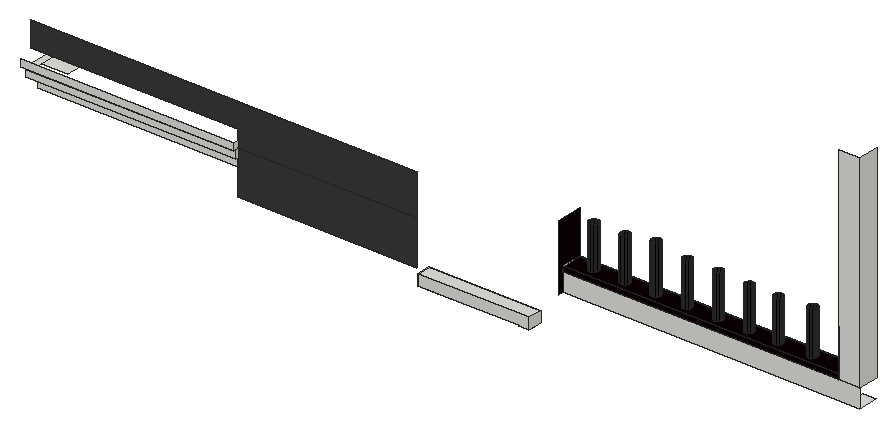
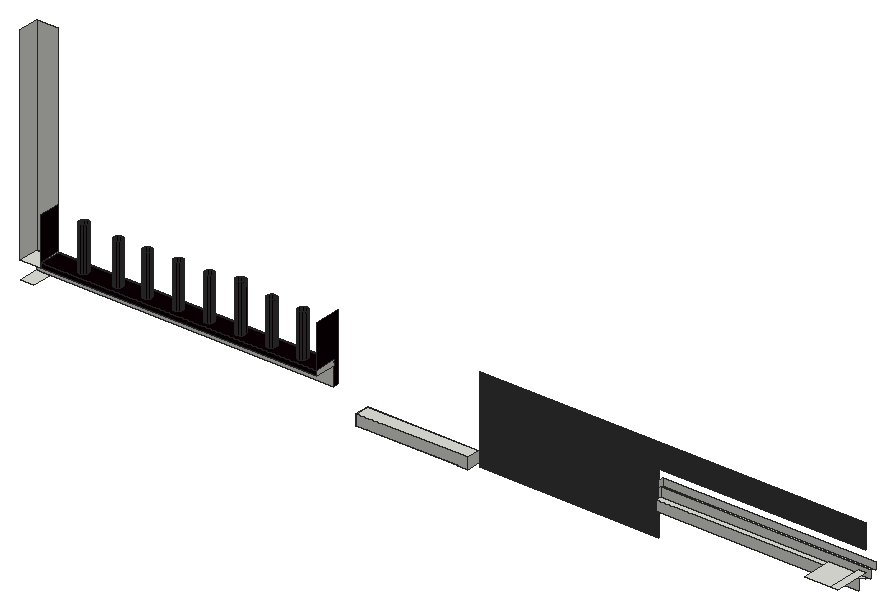
# SketchUp Ruby script. Lengths in inches.
U = 1.inch
M = Sketchup.active_model
def pt(a) = Geom::Point3d.new(a.map { |v| v * U })
def face(e, loops, mat)
  f = e.add_face(loops[0].map { |a| pt(a) })
  loops[1..].each { |l| e.add_face(l.map { |a| pt(a) }).erase! }
  f.material = f.back_material = mat if mat
  f
end
# faces: each face lists its corners as indices into pts; further lists are holes
def faces(e, pts, list, mat = nil) = list.each { |f| face(e, (f[0].is_a?(Array) ? f : [f]).map { |l| l.map { |i| pts[i] } }, mat) }
# xy, xz, yz: faces in a plane at the given z, y or x. An outline is a flat list of corners, or four numbers for a rectangle; further outlines are holes
def ring(l) = l.size == 4 ? [[l[0], l[1]], [l[2], l[1]], [l[2], l[3]], [l[0], l[3]]] : l.each_slice(2).to_a
def flat(e, list, mat, &to3) = list.each { |f| face(e, (f[0].is_a?(Array) ? f : [f]).map { |l| ring(l).map { |u, v| to3.(u, v) } }, mat) }
def xy(e, z, list, mat = nil) = flat(e, list, mat) { |x, y| [x, y, z] }
def xz(e, y, list, mat = nil) = flat(e, list, mat) { |x, z| [x, y, z] }
def yz(e, x, list, mat = nil) = flat(e, list, mat) { |y, z| [x, y, z] }
def lines(e, pts, list) = list.each { |a, b| e.add_line(pt(pts[a]), pt(pts[b])) }
# prism: a flat outline (further loops are holes) pulled along v
def prism(e, loops, v, mat = nil)
  f = face(e, loops, mat); d = Geom::Vector3d.new(v.map { |x| x * U })
  f.pushpull(f.normal.samedirection?(d) ? d.length : -d.length)
end
def box(e, o, s, mat = nil) = prism(e, [[o, [o[0] + s[0], o[1], o[2]], [o[0] + s[0], o[1] + s[1], o[2]], [o[0], o[1] + s[1], o[2]]]], [0, 0, s[2]], mat)
def at(x, y, z, deg = 0) = Geom::Transformation.translation(pt([x, y, z])) * Geom::Transformation.rotation(ORIGIN, Z_AXIS, deg.degrees)
def axes(o, x, y, z) = Geom::Transformation.new([*x, 0, *y, 0, *z, 0, *pt(o).to_a, 1])
def part(name) = M.definitions.add(name)
# library, detail: a bought-in or finely detailed component or shape, given as its bounding box
def library(name, o, s) = part(name).tap { |d| box(d.entities, o, s) }
def detail(e, o, s) = box(e.add_group.entities, o, s)
def put(e, d, t, mat = nil) = e.add_instance(d, t).tap { |i| i.material = mat if mat }
def group(e, t, mat = nil) = e.add_group.tap { |g| g.transformation = t; g.material = mat if mat }.entities
root = M.entities
M.materials.add("[Color M07]").color = [58, 58, 58]
M.materials.add("[Metal Seamed]").color = [11, 0, 4]
xy(root,387.29,[[283.95,58.1,290.34,67.28],[350.03,58.1,357.14,60.85],[291.14,60.85,350.03,67.28],[350.03,60.85,353.83,67.28],[353.83,60.85,357.14,67.28]])
xy(root,387.57,[[290.34,58.1,350.03,67.28]])
xy(root,394.6,[[283.95,58.1,357.14,67.28]])
xy(root,408,[[555.7,70.97,564.5,84.18]])
xy(root,414.75,[[21.75,65.66,21.75,67.28,24.25,67.28,24.25,69.47,158,69.47,158,65.66]])
xy(root,420,[[369.3125,70.97,550.8125,84.66],[550.8125,70.97,564.5,84.66]])
xy(root,420.5,[[21.75,63.91,158,65.66],[19.4375,70.02,24.07,92.83],[24.07,73.08,41.19,92.83]])
xy(root,423.375,[[383.69,75.15,382.92,75.25,382.19,75.55,381.57,76.03,381.09,76.65,380.79,77.37,380.69,78.15,380.79,78.92,381.09,79.65,381.57,80.27,382.19,80.75,382.92,81.05,383.69,81.15,384.47,81.05,385.19,80.75,385.8125,80.27,386.29,79.65,386.59,78.92,386.69,78.15,386.59,77.37,386.29,76.65,385.8125,76.03,385.19,75.55,384.47,75.25],[404.19,75.15,403.42,75.25,402.69,75.55,402.07,76.03,401.59,76.65,401.29,77.37,401.19,78.15,401.29,78.92,401.59,79.65,402.07,80.27,402.69,80.75,403.42,81.05,404.19,81.15,404.97,81.05,405.69,80.75,406.3125,80.27,406.79,79.65,407.09,78.92,407.19,78.15,407.09,77.37,406.79,76.65,406.3125,76.03,405.69,75.55,404.97,75.25],[424.69,75.15,423.92,75.25,423.19,75.55,422.57,76.03,422.09,76.65,421.79,77.37,421.69,78.15,421.79,78.92,422.09,79.65,422.57,80.27,423.19,80.75,423.92,81.05,424.69,81.15,425.47,81.05,426.19,80.75,426.8125,80.27,427.29,79.65,427.59,78.92,427.69,78.15,427.59,77.37,427.29,76.65,426.8125,76.03,426.19,75.55,425.47,75.25],[445.19,75.15,444.42,75.25,443.69,75.55,443.07,76.03,442.59,76.65,442.29,77.37,442.19,78.15,442.29,78.92,442.59,79.65,443.07,80.27,443.69,80.75,444.42,81.05,445.19,81.15,445.97,81.05,446.69,80.75,447.3125,80.27,447.79,79.65,448.09,78.92,448.19,78.15,448.09,77.37,447.79,76.65,447.3125,76.03,446.69,75.55,445.97,75.25],[465.69,75.15,464.92,75.25,464.19,75.55,463.57,76.03,463.09,76.65,462.79,77.37,462.69,78.15,462.79,78.92,463.09,79.65,463.57,80.27,464.19,80.75,464.92,81.05,465.69,81.15,466.47,81.05,467.19,80.75,467.8125,80.27,468.29,79.65,468.59,78.92,468.69,78.15,468.59,77.37,468.29,76.65,467.8125,76.03,467.19,75.55,466.47,75.25],
  [486.19,75.15,485.42,75.25,484.69,75.55,484.07,76.03,483.59,76.65,483.29,77.37,483.19,78.15,483.29,78.92,483.59,79.65,484.07,80.27,484.69,80.75,485.42,81.05,486.19,81.15,486.97,81.05,487.69,80.75,488.3125,80.27,488.79,79.65,489.09,78.92,489.19,78.15,489.09,77.37,488.79,76.65,488.3125,76.03,487.69,75.55,486.97,75.25],[505.19,75.15,504.42,75.25,503.69,75.55,503.07,76.03,502.59,76.65,502.29,77.37,502.19,78.15,502.29,78.92,502.59,79.65,503.07,80.27,503.69,80.75,504.42,81.05,505.19,81.15,505.97,81.05,506.69,80.75,507.3125,80.27,507.79,79.65,508.09,78.92,508.19,78.15,508.09,77.37,507.79,76.65,507.3125,76.03,506.69,75.55,505.97,75.25],[527.82,75.15,527.04,75.25,526.32,75.55,525.7,76.03,525.22,76.65,524.92,77.37,524.82,78.15,524.92,78.92,525.22,79.65,525.7,80.27,526.32,80.75,527.04,81.05,527.82,81.15,528.59,81.05,529.32,80.75,529.9375,80.27,530.42,79.65,530.72,78.92,530.82,78.15,530.72,77.37,530.42,76.65,529.9375,76.03,529.32,75.55,528.59,75.25]])
xy(root,423.375,[[[369.3125,70.97,550.8125,84.66],[383.69,75.15,382.92,75.25,382.19,75.55,381.57,76.03,381.09,76.65,380.79,77.37,380.69,78.15,380.79,78.92,381.09,79.65,381.57,80.27,382.19,80.75,382.92,81.05,383.69,81.15,384.47,81.05,385.19,80.75,385.8125,80.27,386.29,79.65,386.59,78.92,386.69,78.15,386.59,77.37,386.29,76.65,385.8125,76.03,385.19,75.55,384.47,75.25],[404.19,75.15,403.42,75.25,402.69,75.55,402.07,76.03,401.59,76.65,401.29,77.37,401.19,78.15,401.29,78.92,401.59,79.65,402.07,80.27,402.69,80.75,403.42,81.05,404.19,81.15,404.97,81.05,405.69,80.75,406.3125,80.27,406.79,79.65,407.09,78.92,407.19,78.15,407.09,77.37,406.79,76.65,406.3125,76.03,405.69,75.55,404.97,75.25],[424.69,75.15,423.92,75.25,423.19,75.55,422.57,76.03,422.09,76.65,421.79,77.37,421.69,78.15,421.79,78.92,422.09,79.65,422.57,80.27,423.19,80.75,423.92,81.05,424.69,81.15,425.47,81.05,426.19,80.75,426.8125,80.27,427.29,79.65,427.59,78.92,427.69,78.15,427.59,77.37,427.29,76.65,426.8125,76.03,426.19,75.55,425.47,75.25],[445.19,75.15,444.42,75.25,443.69,75.55,443.07,76.03,442.59,76.65,442.29,77.37,442.19,78.15,442.29,78.92,442.59,79.65,443.07,80.27,443.69,80.75,444.42,81.05,445.19,81.15,445.97,81.05,446.69,80.75,447.3125,80.27,447.79,79.65,448.09,78.92,448.19,78.15,448.09,77.37,447.79,76.65,447.3125,76.03,446.69,75.55,445.97,75.25],[465.69,75.15,464.92,75.25,464.19,75.55,463.57,76.03,463.09,76.65,462.79,77.37,462.69,78.15,462.79,78.92,463.09,79.65,463.57,80.27,464.19,80.75,464.92,81.05,465.69,81.15,466.47,81.05,467.19,80.75,467.8125,80.27,468.29,79.65,468.59,78.92,468.69,78.15,468.59,77.37,468.29,76.65,467.8125,76.03,467.19,75.55,466.47,75.25],[486.19,75.15,485.42,75.25,484.69,75.55,484.07,76.03,483.59,76.65,483.29,77.37,483.19,78.15,483.29,78.92,483.59,79.65,484.07,80.27,484.69,80.75,485.42,81.05,486.19,81.15,486.97,81.05,487.69,80.75,488.3125,80.27,488.79,79.65,489.09,78.92,489.19,78.15,489.09,77.37,488.79,76.65,488.3125,76.03,487.69,75.55,486.97,75.25],[505.19,75.15,504.42,75.25,503.69,75.55,503.07,76.03,502.59,76.65,502.29,77.37,502.19,78.15,502.29,78.92,502.59,79.65,503.07,80.27,503.69,80.75,504.42,81.05,505.19,81.15,505.97,81.05,506.69,80.75,507.3125,80.27,507.79,79.65,508.09,78.92,508.19,78.15,508.09,77.37,507.79,76.65,507.3125,76.03,506.69,75.55,505.97,75.25],[527.82,75.15,527.04,75.25,526.32,75.55,525.7,76.03,525.22,76.65,524.92,77.37,524.82,78.15,524.92,78.92,525.22,79.65,525.7,80.27,526.32,80.75,527.04,81.05,527.82,81.15,528.59,81.05,529.32,80.75,529.9375,80.27,530.42,79.65,530.72,78.92,530.82,78.15,530.72,77.37,530.42,76.65,529.9375,76.03,529.32,75.55,528.59,75.25]]],"[Metal Seamed]")
xz(root,58.1,[[283.95,387.29,290.34,387.29,290.34,387.57,350.03,387.57,350.03,387.29,357.14,387.29,357.14,394.6,283.95,394.6]])
xz(root,63.91,[[17.375,420.5,158,425]])
xz(root,65.66,[[19.4375,414.75,158,420.5]])
xz(root,67.28,[[283.95,387.29,283.95,394.6,357.14,394.6,357.14,387.29,350.03,387.29,350.03,387.57,290.34,387.57,290.34,387.29]])
xz(root,67.28,[[158,391.4375,275.92,420.5],[158,420.5,275.92,420.5,275.92,448.0625,21.75,448.0625,21.75,432,158,432]],"[Color M07]")
xz(root,69.47,[[24.25,408,158,414.75]])
xz(root,70.97,[[369.3125,408,564.5,420],[550.8125,420,564.5,555.625]])
xz(root,70.97,[[369.3125,420,550.8125,423.375]],"[Metal Seamed]")
xz(root,84.66,[[369.3125,420,550.8125,423.375]],"[Metal Seamed]")
yz(root,158,[[67.28,408,69.47,414.75],[65.66,414.75,67.28,420.5],[63.91,420.5,67.28,425]])
yz(root,283.95,[[58.1,387.29,67.28,394.6]])
yz(root,290.34,[[58.1,387.29,67.28,387.57]])
yz(root,350.03,[[58.1,387.29,67.28,387.57]])
yz(root,357.14,[[58.1,387.29,67.28,394.6]])
yz(root,369.3125,[[70.97,420,84.66,423.375]])
yz(root,369.3125,[[67.28,408,70.97,408,70.97,423.375,84.66,423.375,84.66,451.5625,67.28,451.5625]],"[Metal Seamed]")
yz(root,550.8125,[[70.97,420,84.66,423.375]])
yz(root,550.8125,[[70.97,423.375,84.66,451.5625]],"[Metal Seamed]")
yz(root,564.5,[[70.97,420,84.66,555.625]])
p = [[382.92,75.25,423.375],[383.69,75.15,423.375],[383.69,75.15,451.5625],[382.92,75.25,451.5625],[384.47,75.25,423.375],[384.47,75.25,451.5625],
  [403.42,75.25,423.375],[404.19,75.15,423.375],[404.19,75.15,451.5625],[403.42,75.25,451.5625],[404.97,75.25,423.375],[404.97,75.25,451.5625],
  [423.92,75.25,423.375],[424.69,75.15,423.375],[424.69,75.15,454.875],[423.92,75.25,454.875],[425.47,75.25,423.375],[425.47,75.25,454.875],
  [444.42,75.25,423.375],[445.19,75.15,423.375],[445.19,75.15,451.5625],[444.42,75.25,451.5625],[445.97,75.25,423.375],[445.97,75.25,451.5625],
  [464.92,75.25,423.375],[465.69,75.15,423.375],[465.69,75.15,451.6875],[464.92,75.25,451.6875],[466.47,75.25,423.375],[466.47,75.25,451.6875],
  [485.42,75.25,423.375],[486.19,75.15,423.375],[486.19,75.15,450.75],[485.42,75.25,450.75],[486.97,75.25,423.375],[486.97,75.25,450.75],
  [504.42,75.25,423.375],[505.19,75.15,423.375],[505.19,75.15,450.5],[504.42,75.25,450.5],[505.97,75.25,423.375],[505.97,75.25,450.5],
  [527.04,75.25,423.375],[527.82,75.15,423.375],[527.82,75.15,452.1875],[527.04,75.25,452.1875],[528.59,75.25,423.375],[528.59,75.25,452.1875],
  [382.19,75.55,423.375],[382.19,75.55,451.5625],[385.19,75.55,423.375],[385.19,75.55,451.5625],[402.69,75.55,423.375],[402.69,75.55,451.5625],
  [405.69,75.55,423.375],[405.69,75.55,451.5625],[423.19,75.55,423.375],[423.19,75.55,454.875],[426.19,75.55,423.375],[426.19,75.55,454.875],
  [443.69,75.55,423.375],[443.69,75.55,451.5625],[446.69,75.55,423.375],[446.69,75.55,451.5625],[464.19,75.55,423.375],[464.19,75.55,451.6875],
  [467.19,75.55,423.375],[467.19,75.55,451.6875],[484.69,75.55,423.375],[484.69,75.55,450.75],[487.69,75.55,423.375],[487.69,75.55,450.75],
  [503.69,75.55,423.375],[503.69,75.55,450.5],[506.69,75.55,423.375],[506.69,75.55,450.5],[526.32,75.55,423.375],[526.32,75.55,452.1875],
  [529.32,75.55,423.375],[529.32,75.55,452.1875],[381.57,76.03,423.375],[381.57,76.03,451.5625],[385.8125,76.03,423.375],[385.8125,76.03,451.5625],
  [402.07,76.03,423.375],[402.07,76.03,451.5625],[406.3125,76.03,423.375],[406.3125,76.03,451.5625],[422.57,76.03,423.375],[422.57,76.03,454.875],
  [426.8125,76.03,423.375],[426.8125,76.03,454.875],[443.07,76.03,423.375],[443.07,76.03,451.5625],[447.3125,76.03,423.375],[447.3125,76.03,451.5625],
  [463.57,76.03,423.375],[463.57,76.03,451.6875],[467.8125,76.03,423.375],[467.8125,76.03,451.6875],[484.07,76.03,423.375],[484.07,76.03,450.75],
  [488.3125,76.03,423.375],[488.3125,76.03,450.75],[503.07,76.03,423.375],[503.07,76.03,450.5],[507.3125,76.03,423.375],[507.3125,76.03,450.5],
  [525.7,76.03,423.375],[525.7,76.03,452.1875],[529.9375,76.03,423.375],[529.9375,76.03,452.1875],[381.09,76.65,423.375],[381.09,76.65,451.5625],
  [386.29,76.65,423.375],[386.29,76.65,451.5625],[401.59,76.65,423.375],[401.59,76.65,451.5625],[406.79,76.65,423.375],[406.79,76.65,451.5625],
  [422.09,76.65,423.375],[422.09,76.65,454.875],[427.29,76.65,423.375],[427.29,76.65,454.875],[442.59,76.65,423.375],[442.59,76.65,451.5625],
  [447.79,76.65,423.375],[447.79,76.65,451.5625],[463.09,76.65,423.375],[463.09,76.65,451.6875],[468.29,76.65,423.375],[468.29,76.65,451.6875],
  [483.59,76.65,423.375],[483.59,76.65,450.75],[488.79,76.65,423.375],[488.79,76.65,450.75],[502.59,76.65,423.375],[502.59,76.65,450.5],
  [507.79,76.65,423.375],[507.79,76.65,450.5],[525.22,76.65,423.375],[525.22,76.65,452.1875],[530.42,76.65,423.375],[530.42,76.65,452.1875],
  [380.79,77.37,423.375],[380.79,77.37,451.5625],[386.59,77.37,423.375],[386.59,77.37,451.5625],[401.29,77.37,423.375],[401.29,77.37,451.5625],
  [407.09,77.37,423.375],[407.09,77.37,451.5625],[421.79,77.37,423.375],[421.79,77.37,454.875],[427.59,77.37,423.375],[427.59,77.37,454.875],
  [442.29,77.37,423.375],[442.29,77.37,451.5625],[448.09,77.37,423.375],[448.09,77.37,451.5625],[462.79,77.37,423.375],[462.79,77.37,451.6875],
  [468.59,77.37,423.375],[468.59,77.37,451.6875],[483.29,77.37,423.375],[483.29,77.37,450.75],[489.09,77.37,423.375],[489.09,77.37,450.75],
  [502.29,77.37,423.375],[502.29,77.37,450.5],[508.09,77.37,423.375],[508.09,77.37,450.5],[524.92,77.37,423.375],[524.92,77.37,452.1875],
  [530.72,77.37,423.375],[530.72,77.37,452.1875],[380.69,78.15,423.375],[380.69,78.15,451.5625],[386.69,78.15,423.375],[386.69,78.15,451.5625],
  [401.19,78.15,423.375],[401.19,78.15,451.5625],[407.19,78.15,423.375],[407.19,78.15,451.5625],[421.69,78.15,423.375],[421.69,78.15,454.875],
  [427.69,78.15,423.375],[427.69,78.15,454.875],[442.19,78.15,423.375],[442.19,78.15,451.5625],[448.19,78.15,423.375],[448.19,78.15,451.5625],
  [462.69,78.15,423.375],[462.69,78.15,451.6875],[468.69,78.15,423.375],[468.69,78.15,451.6875],[483.19,78.15,423.375],[483.19,78.15,450.75],
  [489.19,78.15,423.375],[489.19,78.15,450.75],[502.19,78.15,423.375],[502.19,78.15,450.5],[508.19,78.15,423.375],[508.19,78.15,450.5],
  [524.82,78.15,423.375],[524.82,78.15,452.1875],[530.82,78.15,423.375],[530.82,78.15,452.1875],[380.79,78.92,423.375],[380.79,78.92,451.5625],
  [386.59,78.92,423.375],[386.59,78.92,451.5625],[401.29,78.92,423.375],[401.29,78.92,451.5625],[407.09,78.92,423.375],[407.09,78.92,451.5625],
  [421.79,78.92,423.375],[421.79,78.92,454.875],[427.59,78.92,423.375],[427.59,78.92,454.875],[442.29,78.92,423.375],[442.29,78.92,451.5625],
  [448.09,78.92,423.375],[448.09,78.92,451.5625],[462.79,78.92,423.375],[462.79,78.92,451.6875],[468.59,78.92,423.375],[468.59,78.92,451.6875],
  [483.29,78.92,423.375],[483.29,78.92,450.75],[489.09,78.92,423.375],[489.09,78.92,450.75],[502.29,78.92,423.375],[502.29,78.92,450.5],
  [508.09,78.92,423.375],[508.09,78.92,450.5],[524.92,78.92,423.375],[524.92,78.92,452.1875],[530.72,78.92,423.375],[530.72,78.92,452.1875],
  [381.09,79.65,423.375],[381.09,79.65,451.5625],[386.29,79.65,423.375],[386.29,79.65,451.5625],[401.59,79.65,423.375],[401.59,79.65,451.5625],
  [406.79,79.65,423.375],[406.79,79.65,451.5625],[422.09,79.65,423.375],[422.09,79.65,454.875],[427.29,79.65,423.375],[427.29,79.65,454.875],
  [442.59,79.65,423.375],[442.59,79.65,451.5625],[447.79,79.65,423.375],[447.79,79.65,451.5625],[463.09,79.65,423.375],[463.09,79.65,451.6875],
  [468.29,79.65,423.375],[468.29,79.65,451.6875],[483.59,79.65,423.375],[483.59,79.65,450.75],[488.79,79.65,423.375],[488.79,79.65,450.75],
  [502.59,79.65,423.375],[502.59,79.65,450.5],[507.79,79.65,423.375],[507.79,79.65,450.5],[525.22,79.65,423.375],[525.22,79.65,452.1875],
  [530.42,79.65,423.375],[530.42,79.65,452.1875],[381.57,80.27,423.375],[381.57,80.27,451.5625],[385.8125,80.27,423.375],[385.8125,80.27,451.5625],
  [402.07,80.27,423.375],[402.07,80.27,451.5625],[406.3125,80.27,423.375],[406.3125,80.27,451.5625],[422.57,80.27,423.375],[422.57,80.27,454.875],
  [426.8125,80.27,423.375],[426.8125,80.27,454.875],[443.07,80.27,423.375],[443.07,80.27,451.5625],[447.3125,80.27,423.375],[447.3125,80.27,451.5625],
  [463.57,80.27,423.375],[463.57,80.27,451.6875],[467.8125,80.27,423.375],[467.8125,80.27,451.6875],[484.07,80.27,423.375],[484.07,80.27,450.75],
  [488.3125,80.27,423.375],[488.3125,80.27,450.75],[503.07,80.27,423.375],[503.07,80.27,450.5],[507.3125,80.27,423.375],[507.3125,80.27,450.5],
  [525.7,80.27,423.375],[525.7,80.27,452.1875],[529.9375,80.27,423.375],[529.9375,80.27,452.1875],[382.19,80.75,423.375],[382.19,80.75,451.5625],
  [385.19,80.75,423.375],[385.19,80.75,451.5625],[402.69,80.75,423.375],[402.69,80.75,451.5625],[405.69,80.75,423.375],[405.69,80.75,451.5625],
  [423.19,80.75,423.375],[423.19,80.75,454.875],[426.19,80.75,423.375],[426.19,80.75,454.875],[443.69,80.75,423.375],[443.69,80.75,451.5625],
  [446.69,80.75,423.375],[446.69,80.75,451.5625],[464.19,80.75,423.375],[464.19,80.75,451.6875],[467.19,80.75,423.375],[467.19,80.75,451.6875],
  [484.69,80.75,423.375],[484.69,80.75,450.75],[487.69,80.75,423.375],[487.69,80.75,450.75],[503.69,80.75,423.375],[503.69,80.75,450.5],
  [506.69,80.75,423.375],[506.69,80.75,450.5],[526.32,80.75,423.375],[526.32,80.75,452.1875],[529.32,80.75,423.375],[529.32,80.75,452.1875],
  [382.92,81.05,423.375],[382.92,81.05,451.5625],[384.47,81.05,423.375],[384.47,81.05,451.5625],[403.42,81.05,423.375],[403.42,81.05,451.5625],
  [404.97,81.05,423.375],[404.97,81.05,451.5625],[423.92,81.05,423.375],[423.92,81.05,454.875],[425.47,81.05,423.375],[425.47,81.05,454.875],
  [444.42,81.05,423.375],[444.42,81.05,451.5625],[445.97,81.05,423.375],[445.97,81.05,451.5625],[464.92,81.05,423.375],[464.92,81.05,451.6875],
  [466.47,81.05,423.375],[466.47,81.05,451.6875],[485.42,81.05,423.375],[485.42,81.05,450.75],[486.97,81.05,423.375],[486.97,81.05,450.75],
  [504.42,81.05,423.375],[504.42,81.05,450.5],[505.97,81.05,423.375],[505.97,81.05,450.5],[527.04,81.05,423.375],[527.04,81.05,452.1875],
  [528.59,81.05,423.375],[528.59,81.05,452.1875],[383.69,81.15,423.375],[383.69,81.15,451.5625],[404.19,81.15,423.375],[404.19,81.15,451.5625],
  [424.69,81.15,423.375],[424.69,81.15,454.875],[445.19,81.15,423.375],[445.19,81.15,451.5625],[465.69,81.15,423.375],[465.69,81.15,451.6875],
  [486.19,81.15,423.375],[486.19,81.15,450.75],[505.19,81.15,423.375],[505.19,81.15,450.5],[527.82,81.15,423.375],[527.82,81.15,452.1875]]
faces(root,p,[[0,1,2,3],[1,4,5,2],[6,7,8,9],[7,10,11,8],[12,13,14,15],[13,16,17,14],[18,19,20,21],[19,22,23,20],
  [24,25,26,27],[25,28,29,26],[30,31,32,33],[31,34,35,32],[36,37,38,39],[37,40,41,38],[42,43,44,45],[43,46,47,44],
  [48,0,3,49],[4,50,51,5],[52,6,9,53],[10,54,55,11],[56,12,15,57],[16,58,59,17],[60,18,21,61],[22,62,63,23],
  [64,24,27,65],[28,66,67,29],[68,30,33,69],[34,70,71,35],[72,36,39,73],[40,74,75,41],[76,42,45,77],[46,78,79,47],
  [80,48,49,81],[50,82,83,51],[84,52,53,85],[54,86,87,55],[88,56,57,89],[58,90,91,59],[92,60,61,93],[62,94,95,63],
  [96,64,65,97],[66,98,99,67],[100,68,69,101],[70,102,103,71],[104,72,73,105],[74,106,107,75],[108,76,77,109],[78,110,111,79],
  [112,80,81,113],[82,114,115,83],[116,84,85,117],[86,118,119,87],[120,88,89,121],[90,122,123,91],[124,92,93,125],[94,126,127,95],
  [128,96,97,129],[98,130,131,99],[132,100,101,133],[102,134,135,103],[136,104,105,137],[106,138,139,107],[140,108,109,141],[110,142,143,111],
  [144,112,113,145],[114,146,147,115],[148,116,117,149],[118,150,151,119],[152,120,121,153],[122,154,155,123],[156,124,125,157],[126,158,159,127],
  [160,128,129,161],[130,162,163,131],[164,132,133,165],[134,166,167,135],[168,136,137,169],[138,170,171,139],[172,140,141,173],[142,174,175,143],
  [176,144,145,177],[146,178,179,147],[180,148,149,181],[150,182,183,151],[184,152,153,185],[154,186,187,155],[188,156,157,189],[158,190,191,159],
  [192,160,161,193],[162,194,195,163],[196,164,165,197],[166,198,199,167],[200,168,169,201],[170,202,203,171],[204,172,173,205],[174,206,207,175],
  [208,176,177,209],[178,210,211,179],[212,180,181,213],[182,214,215,183],[216,184,185,217],[186,218,219,187],[220,188,189,221],[190,222,223,191],
  [224,192,193,225],[194,226,227,195],[228,196,197,229],[198,230,231,199],[232,200,201,233],[202,234,235,203],[236,204,205,237],[206,238,239,207],
  [240,208,209,241],[210,242,243,211],[244,212,213,245],[214,246,247,215],[248,216,217,249],[218,250,251,219],[252,220,221,253],[222,254,255,223],
  [256,224,225,257],[226,258,259,227],[260,228,229,261],[230,262,263,231],[264,232,233,265],[234,266,267,235],[268,236,237,269],[238,270,271,239],
  [272,240,241,273],[242,274,275,243],[276,244,245,277],[246,278,279,247],[280,248,249,281],[250,282,283,251],[284,252,253,285],[254,286,287,255],
  [288,256,257,289],[258,290,291,259],[292,260,261,293],[262,294,295,263],[296,264,265,297],[266,298,299,267],[300,268,269,301],[270,302,303,271],
  [304,272,273,305],[274,306,307,275],[308,276,277,309],[278,310,311,279],[312,280,281,313],[282,314,315,283],[316,284,285,317],[286,318,319,287],
  [320,288,289,321],[290,322,323,291],[324,292,293,325],[294,326,327,295],[328,296,297,329],[298,330,331,299],[332,300,301,333],[302,334,335,303],
  [336,304,305,337],[306,338,339,307],[340,308,309,341],[310,342,343,311],[344,312,313,345],[314,346,347,315],[348,316,317,349],[318,350,351,319],
  [352,320,321,353],[322,354,355,323],[356,324,325,357],[326,358,359,327],[360,328,329,361],[330,362,363,331],[364,332,333,365],[334,366,367,335],
  [368,336,337,369],[338,368,369,339],[370,340,341,371],[342,370,371,343],[372,344,345,373],[346,372,373,347],[374,348,349,375],[350,374,375,351],
  [376,352,353,377],[354,376,377,355],[378,356,357,379],[358,378,379,359],[380,360,361,381],[362,380,381,363],[382,364,365,383],[366,382,383,367]],"[Metal Seamed]")
